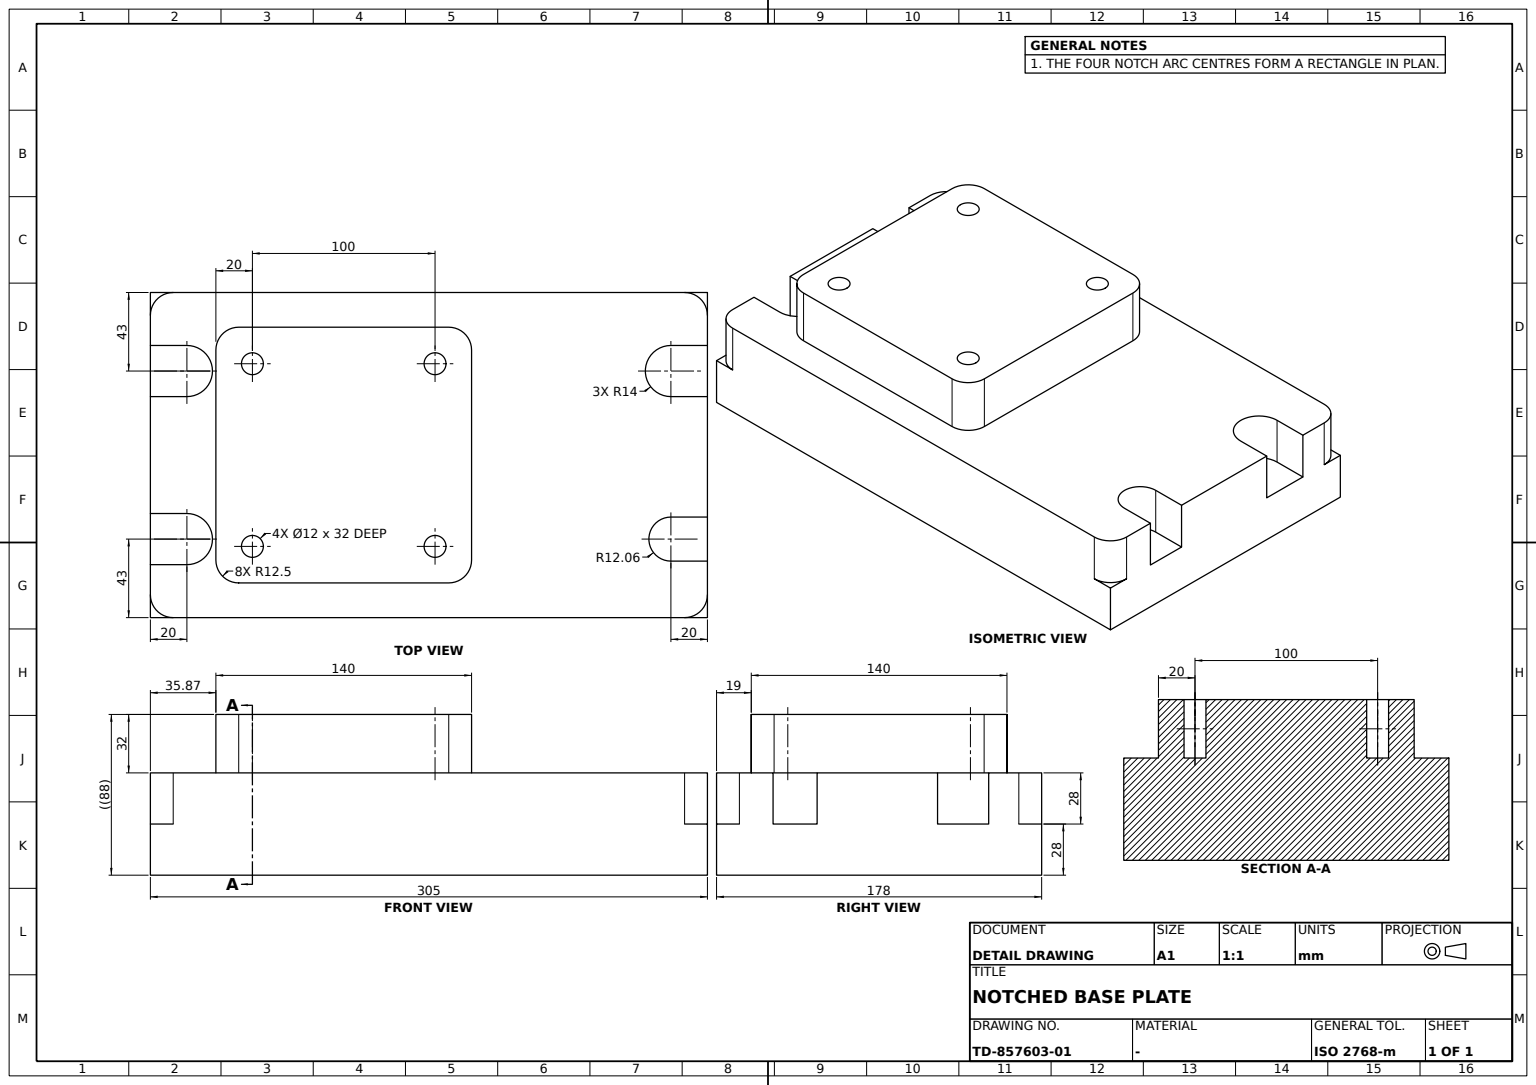
ISO-10303-21;
HEADER;
FILE_DESCRIPTION((''),'2;1');
FILE_NAME('','',(''),(''),'','','');
FILE_SCHEMA(('AUTOMOTIVE_DESIGN'));
ENDSEC;
DATA;
#1=APPLICATION_CONTEXT('');
#2=PRODUCT_CONTEXT('',#1,'mechanical');
#3=PRODUCT('','','',(#2));
#4=PRODUCT_DEFINITION_FORMATION('','',#3);
#5=PRODUCT_DEFINITION_CONTEXT('',#1,'design');
#6=PRODUCT_DEFINITION('','',#4,#5);
#7=PRODUCT_DEFINITION_SHAPE('','',#6);
#8=(LENGTH_UNIT()NAMED_UNIT(*)SI_UNIT(.MILLI.,.METRE.));
#9=(NAMED_UNIT(*)PLANE_ANGLE_UNIT()SI_UNIT($,.RADIAN.));
#10=(NAMED_UNIT(*)SI_UNIT($,.STERADIAN.)SOLID_ANGLE_UNIT());
#11=UNCERTAINTY_MEASURE_WITH_UNIT(LENGTH_MEASURE(1.E-05),#8,'distance_accuracy_value','');
#12=(GEOMETRIC_REPRESENTATION_CONTEXT(3)GLOBAL_UNCERTAINTY_ASSIGNED_CONTEXT((#11))GLOBAL_UNIT_ASSIGNED_CONTEXT((#8,#9,#10))REPRESENTATION_CONTEXT('',''));
#13=CARTESIAN_POINT('',(44.,50.,0.));
#14=VERTEX_POINT('',#13);
#15=CARTESIAN_POINT('',(56.,50.,0.));
#16=VERTEX_POINT('',#15);
#17=CARTESIAN_POINT('',(50.,50.,0.));
#18=DIRECTION('',(0.,0.,1.));
#19=DIRECTION('',(1.,0.,0.));
#20=AXIS2_PLACEMENT_3D('',#17,#18,#19);
#21=CIRCLE('',#20,6.);
#22=EDGE_CURVE('',#14,#16,#21,.T.);
#23=ORIENTED_EDGE('',*,*,#22,.F.);
#24=CARTESIAN_POINT('',(44.,50.,32.));
#25=VERTEX_POINT('',#24);
#26=CARTESIAN_POINT('',(44.,50.,16.));
#27=VECTOR('',#18,1000.);
#28=LINE('',#26,#27);
#29=EDGE_CURVE('',#14,#25,#28,.T.);
#30=ORIENTED_EDGE('',*,*,#29,.T.);
#31=CARTESIAN_POINT('',(56.,50.,32.));
#32=VERTEX_POINT('',#31);
#33=CARTESIAN_POINT('',(50.,50.,32.));
#34=AXIS2_PLACEMENT_3D('',#33,#18,#19);
#35=CIRCLE('',#34,6.);
#36=EDGE_CURVE('',#25,#32,#35,.T.);
#37=ORIENTED_EDGE('',*,*,#36,.T.);
#38=CARTESIAN_POINT('',(56.,50.,16.));
#39=LINE('',#38,#27);
#40=EDGE_CURVE('',#16,#32,#39,.T.);
#41=ORIENTED_EDGE('',*,*,#40,.F.);
#42=EDGE_LOOP('',(#23,#30,#37,#41));
#43=FACE_OUTER_BOUND('',#42,.T.);
#44=CARTESIAN_POINT('',(50.,50.,16.));
#45=DIRECTION('',(0.,0.,-1.));
#46=AXIS2_PLACEMENT_3D('',#44,#45,#19);
#47=CYLINDRICAL_SURFACE('',#46,6.);
#48=ADVANCED_FACE('',(#43),#47,.F.);
#49=EDGE_CURVE('',#16,#14,#21,.T.);
#50=ORIENTED_EDGE('',*,*,#49,.T.);
#51=ORIENTED_EDGE('',*,*,#22,.T.);
#52=EDGE_LOOP('',(#50,#51));
#53=FACE_BOUND('',#52,.T.);
#54=CARTESIAN_POINT('',(44.,-50.,0.));
#55=VERTEX_POINT('',#54);
#56=CARTESIAN_POINT('',(56.,-50.,0.));
#57=VERTEX_POINT('',#56);
#58=CARTESIAN_POINT('',(50.,-50.,0.));
#59=AXIS2_PLACEMENT_3D('',#58,#18,#19);
#60=CIRCLE('',#59,6.);
#61=EDGE_CURVE('',#55,#57,#60,.T.);
#62=ORIENTED_EDGE('',*,*,#61,.T.);
#63=EDGE_CURVE('',#57,#55,#60,.T.);
#64=ORIENTED_EDGE('',*,*,#63,.T.);
#65=EDGE_LOOP('',(#62,#64));
#66=FACE_BOUND('',#65,.T.);
#67=CARTESIAN_POINT('',(-44.,-50.,0.));
#68=VERTEX_POINT('',#67);
#69=CARTESIAN_POINT('',(-56.,-50.,0.));
#70=VERTEX_POINT('',#69);
#71=CARTESIAN_POINT('',(-50.,-50.,0.));
#72=AXIS2_PLACEMENT_3D('',#71,#18,#19);
#73=CIRCLE('',#72,6.);
#74=EDGE_CURVE('',#68,#70,#73,.T.);
#75=ORIENTED_EDGE('',*,*,#74,.T.);
#76=EDGE_CURVE('',#70,#68,#73,.T.);
#77=ORIENTED_EDGE('',*,*,#76,.T.);
#78=EDGE_LOOP('',(#75,#77));
#79=FACE_BOUND('',#78,.T.);
#80=CARTESIAN_POINT('',(-46.,0.,0.));
#81=VERTEX_POINT('',#80);
#82=CARTESIAN_POINT('',(46.,0.,0.));
#83=VERTEX_POINT('',#82);
#84=CARTESIAN_POINT('',(0.,0.,0.));
#85=AXIS2_PLACEMENT_3D('',#84,#18,#19);
#86=CIRCLE('',#85,46.);
#87=EDGE_CURVE('',#81,#83,#86,.T.);
#88=ORIENTED_EDGE('',*,*,#87,.T.);
#89=EDGE_CURVE('',#83,#81,#86,.T.);
#90=ORIENTED_EDGE('',*,*,#89,.T.);
#91=EDGE_LOOP('',(#88,#90));
#92=FACE_BOUND('',#91,.T.);
#93=CARTESIAN_POINT('',(-70.,57.5,0.));
#94=VERTEX_POINT('',#93);
#95=CARTESIAN_POINT('',(-70.,-57.5,0.));
#96=VERTEX_POINT('',#95);
#97=CARTESIAN_POINT('',(-70.,0.,0.));
#98=DIRECTION('',(0.,-1.,0.));
#99=VECTOR('',#98,1000.);
#100=LINE('',#97,#99);
#101=EDGE_CURVE('',#94,#96,#100,.T.);
#102=ORIENTED_EDGE('',*,*,#101,.F.);
#103=CARTESIAN_POINT('',(-57.5,70.,0.));
#104=VERTEX_POINT('',#103);
#105=CARTESIAN_POINT('',(-57.5,57.5,0.));
#106=AXIS2_PLACEMENT_3D('',#105,#18,#19);
#107=CIRCLE('',#106,12.5);
#108=EDGE_CURVE('',#104,#94,#107,.T.);
#109=ORIENTED_EDGE('',*,*,#108,.F.);
#110=CARTESIAN_POINT('',(57.5,70.,0.));
#111=VERTEX_POINT('',#110);
#112=CARTESIAN_POINT('',(0.,70.,0.));
#113=DIRECTION('',(-1.,0.,0.));
#114=VECTOR('',#113,1000.);
#115=LINE('',#112,#114);
#116=EDGE_CURVE('',#111,#104,#115,.T.);
#117=ORIENTED_EDGE('',*,*,#116,.F.);
#118=CARTESIAN_POINT('',(70.,57.5,0.));
#119=VERTEX_POINT('',#118);
#120=CARTESIAN_POINT('',(57.5,57.5,0.));
#121=AXIS2_PLACEMENT_3D('',#120,#18,#19);
#122=CIRCLE('',#121,12.5);
#123=EDGE_CURVE('',#119,#111,#122,.T.);
#124=ORIENTED_EDGE('',*,*,#123,.F.);
#125=CARTESIAN_POINT('',(70.,-57.5,0.));
#126=VERTEX_POINT('',#125);
#127=CARTESIAN_POINT('',(70.,0.,0.));
#128=DIRECTION('',(0.,1.,0.));
#129=VECTOR('',#128,1000.);
#130=LINE('',#127,#129);
#131=EDGE_CURVE('',#126,#119,#130,.T.);
#132=ORIENTED_EDGE('',*,*,#131,.F.);
#133=CARTESIAN_POINT('',(57.5,-70.,0.));
#134=VERTEX_POINT('',#133);
#135=CARTESIAN_POINT('',(57.5,-57.5,0.));
#136=AXIS2_PLACEMENT_3D('',#135,#18,#19);
#137=CIRCLE('',#136,12.5);
#138=EDGE_CURVE('',#134,#126,#137,.T.);
#139=ORIENTED_EDGE('',*,*,#138,.F.);
#140=CARTESIAN_POINT('',(-57.5,-70.,0.));
#141=VERTEX_POINT('',#140);
#142=CARTESIAN_POINT('',(0.,-70.,0.));
#143=VECTOR('',#19,1000.);
#144=LINE('',#142,#143);
#145=EDGE_CURVE('',#141,#134,#144,.T.);
#146=ORIENTED_EDGE('',*,*,#145,.F.);
#147=CARTESIAN_POINT('',(-57.5,-57.5,0.));
#148=AXIS2_PLACEMENT_3D('',#147,#18,#19);
#149=CIRCLE('',#148,12.5);
#150=EDGE_CURVE('',#96,#141,#149,.T.);
#151=ORIENTED_EDGE('',*,*,#150,.F.);
#152=EDGE_LOOP('',(#102,#109,#117,#124,#132,#139,#146,#151));
#153=FACE_OUTER_BOUND('',#152,.T.);
#154=CARTESIAN_POINT('',(-44.,50.,0.));
#155=VERTEX_POINT('',#154);
#156=CARTESIAN_POINT('',(-56.,50.,0.));
#157=VERTEX_POINT('',#156);
#158=CARTESIAN_POINT('',(-50.,50.,0.));
#159=AXIS2_PLACEMENT_3D('',#158,#18,#19);
#160=CIRCLE('',#159,6.);
#161=EDGE_CURVE('',#155,#157,#160,.T.);
#162=ORIENTED_EDGE('',*,*,#161,.T.);
#163=EDGE_CURVE('',#157,#155,#160,.T.);
#164=ORIENTED_EDGE('',*,*,#163,.T.);
#165=EDGE_LOOP('',(#162,#164));
#166=FACE_BOUND('',#165,.T.);
#167=PLANE('',#85);
#168=ADVANCED_FACE('',(#53,#66,#79,#92,#153,#166),#167,.F.);
#169=CARTESIAN_POINT('',(57.5,-70.,32.));
#170=VERTEX_POINT('',#169);
#171=CARTESIAN_POINT('',(57.5,-70.,16.));
#172=LINE('',#171,#27);
#173=EDGE_CURVE('',#134,#170,#172,.T.);
#174=ORIENTED_EDGE('',*,*,#173,.T.);
#175=CARTESIAN_POINT('',(-57.5,-70.,32.));
#176=VERTEX_POINT('',#175);
#177=CARTESIAN_POINT('',(0.,-70.,32.));
#178=LINE('',#177,#143);
#179=EDGE_CURVE('',#176,#170,#178,.T.);
#180=ORIENTED_EDGE('',*,*,#179,.F.);
#181=CARTESIAN_POINT('',(-57.5,-70.,16.));
#182=LINE('',#181,#27);
#183=EDGE_CURVE('',#141,#176,#182,.T.);
#184=ORIENTED_EDGE('',*,*,#183,.F.);
#185=ORIENTED_EDGE('',*,*,#145,.T.);
#186=EDGE_LOOP('',(#174,#180,#184,#185));
#187=FACE_OUTER_BOUND('',#186,.T.);
#188=CARTESIAN_POINT('',(70.,-70.,0.));
#189=AXIS2_PLACEMENT_3D('',#188,#128,#113);
#190=PLANE('',#189);
#191=ADVANCED_FACE('',(#187),#190,.F.);
#192=ORIENTED_EDGE('',*,*,#74,.F.);
#193=CARTESIAN_POINT('',(-44.,-50.,32.));
#194=VERTEX_POINT('',#193);
#195=CARTESIAN_POINT('',(-44.,-50.,16.));
#196=LINE('',#195,#27);
#197=EDGE_CURVE('',#68,#194,#196,.T.);
#198=ORIENTED_EDGE('',*,*,#197,.T.);
#199=CARTESIAN_POINT('',(-56.,-50.,32.));
#200=VERTEX_POINT('',#199);
#201=CARTESIAN_POINT('',(-50.,-50.,32.));
#202=AXIS2_PLACEMENT_3D('',#201,#18,#19);
#203=CIRCLE('',#202,6.);
#204=EDGE_CURVE('',#194,#200,#203,.T.);
#205=ORIENTED_EDGE('',*,*,#204,.T.);
#206=CARTESIAN_POINT('',(-56.,-50.,16.));
#207=LINE('',#206,#27);
#208=EDGE_CURVE('',#70,#200,#207,.T.);
#209=ORIENTED_EDGE('',*,*,#208,.F.);
#210=EDGE_LOOP('',(#192,#198,#205,#209));
#211=FACE_OUTER_BOUND('',#210,.T.);
#212=CARTESIAN_POINT('',(-50.,-50.,16.));
#213=AXIS2_PLACEMENT_3D('',#212,#45,#19);
#214=CYLINDRICAL_SURFACE('',#213,6.);
#215=ADVANCED_FACE('',(#211),#214,.F.);
#216=CARTESIAN_POINT('',(70.,-57.5,32.));
#217=VERTEX_POINT('',#216);
#218=CARTESIAN_POINT('',(57.5,-57.5,32.));
#219=AXIS2_PLACEMENT_3D('',#218,#45,#19);
#220=CIRCLE('',#219,12.5);
#221=EDGE_CURVE('',#217,#170,#220,.T.);
#222=ORIENTED_EDGE('',*,*,#221,.T.);
#223=ORIENTED_EDGE('',*,*,#173,.F.);
#224=ORIENTED_EDGE('',*,*,#138,.T.);
#225=CARTESIAN_POINT('',(70.,-57.5,16.));
#226=LINE('',#225,#27);
#227=EDGE_CURVE('',#126,#217,#226,.T.);
#228=ORIENTED_EDGE('',*,*,#227,.T.);
#229=EDGE_LOOP('',(#222,#223,#224,#228));
#230=FACE_OUTER_BOUND('',#229,.T.);
#231=CARTESIAN_POINT('',(57.5,-57.5,16.));
#232=AXIS2_PLACEMENT_3D('',#231,#45,#19);
#233=CYLINDRICAL_SURFACE('',#232,12.5);
#234=ADVANCED_FACE('',(#230),#233,.T.);
#235=ORIENTED_EDGE('',*,*,#101,.T.);
#236=CARTESIAN_POINT('',(-70.,-57.5,32.));
#237=VERTEX_POINT('',#236);
#238=CARTESIAN_POINT('',(-70.,-57.5,16.));
#239=LINE('',#238,#27);
#240=EDGE_CURVE('',#96,#237,#239,.T.);
#241=ORIENTED_EDGE('',*,*,#240,.T.);
#242=CARTESIAN_POINT('',(-70.,57.5,32.));
#243=VERTEX_POINT('',#242);
#244=CARTESIAN_POINT('',(-70.,0.,32.));
#245=LINE('',#244,#99);
#246=EDGE_CURVE('',#243,#237,#245,.T.);
#247=ORIENTED_EDGE('',*,*,#246,.F.);
#248=CARTESIAN_POINT('',(-70.,57.5,16.));
#249=LINE('',#248,#27);
#250=EDGE_CURVE('',#94,#243,#249,.T.);
#251=ORIENTED_EDGE('',*,*,#250,.F.);
#252=EDGE_LOOP('',(#235,#241,#247,#251));
#253=FACE_OUTER_BOUND('',#252,.T.);
#254=CARTESIAN_POINT('',(-70.,70.,0.));
#255=AXIS2_PLACEMENT_3D('',#254,#113,#98);
#256=PLANE('',#255);
#257=ADVANCED_FACE('',(#253),#256,.T.);
#258=EDGE_CURVE('',#32,#25,#35,.T.);
#259=ORIENTED_EDGE('',*,*,#258,.T.);
#260=ORIENTED_EDGE('',*,*,#29,.F.);
#261=ORIENTED_EDGE('',*,*,#49,.F.);
#262=ORIENTED_EDGE('',*,*,#40,.T.);
#263=EDGE_LOOP('',(#259,#260,#261,#262));
#264=FACE_OUTER_BOUND('',#263,.T.);
#265=ADVANCED_FACE('',(#264),#47,.F.);
#266=CARTESIAN_POINT('',(44.,-50.,32.));
#267=VERTEX_POINT('',#266);
#268=CARTESIAN_POINT('',(44.,-50.,16.));
#269=LINE('',#268,#27);
#270=EDGE_CURVE('',#55,#267,#269,.T.);
#271=ORIENTED_EDGE('',*,*,#270,.F.);
#272=ORIENTED_EDGE('',*,*,#63,.F.);
#273=CARTESIAN_POINT('',(56.,-50.,32.));
#274=VERTEX_POINT('',#273);
#275=CARTESIAN_POINT('',(56.,-50.,16.));
#276=LINE('',#275,#27);
#277=EDGE_CURVE('',#57,#274,#276,.T.);
#278=ORIENTED_EDGE('',*,*,#277,.T.);
#279=CARTESIAN_POINT('',(50.,-50.,32.));
#280=AXIS2_PLACEMENT_3D('',#279,#18,#19);
#281=CIRCLE('',#280,6.);
#282=EDGE_CURVE('',#274,#267,#281,.T.);
#283=ORIENTED_EDGE('',*,*,#282,.T.);
#284=EDGE_LOOP('',(#271,#272,#278,#283));
#285=FACE_OUTER_BOUND('',#284,.T.);
#286=CARTESIAN_POINT('',(50.,-50.,16.));
#287=AXIS2_PLACEMENT_3D('',#286,#45,#19);
#288=CYLINDRICAL_SURFACE('',#287,6.);
#289=ADVANCED_FACE('',(#285),#288,.F.);
#290=CARTESIAN_POINT('',(-46.,0.,32.));
#291=VERTEX_POINT('',#290);
#292=CARTESIAN_POINT('',(-46.,0.,15.34));
#293=VECTOR('',#45,1000.);
#294=LINE('',#292,#293);
#295=EDGE_CURVE('',#291,#81,#294,.T.);
#296=ORIENTED_EDGE('',*,*,#295,.T.);
#297=ORIENTED_EDGE('',*,*,#89,.F.);
#298=CARTESIAN_POINT('',(46.,0.,32.));
#299=VERTEX_POINT('',#298);
#300=CARTESIAN_POINT('',(46.,0.,15.34));
#301=LINE('',#300,#293);
#302=EDGE_CURVE('',#299,#83,#301,.T.);
#303=ORIENTED_EDGE('',*,*,#302,.F.);
#304=CARTESIAN_POINT('',(0.,0.,32.));
#305=AXIS2_PLACEMENT_3D('',#304,#18,#19);
#306=CIRCLE('',#305,46.);
#307=EDGE_CURVE('',#299,#291,#306,.T.);
#308=ORIENTED_EDGE('',*,*,#307,.T.);
#309=EDGE_LOOP('',(#296,#297,#303,#308));
#310=FACE_OUTER_BOUND('',#309,.T.);
#311=CARTESIAN_POINT('',(0.,0.,15.34));
#312=AXIS2_PLACEMENT_3D('',#311,#45,#19);
#313=CYLINDRICAL_SURFACE('',#312,46.);
#314=ADVANCED_FACE('',(#310),#313,.F.);
#315=ORIENTED_EDGE('',*,*,#61,.F.);
#316=ORIENTED_EDGE('',*,*,#270,.T.);
#317=EDGE_CURVE('',#267,#274,#281,.T.);
#318=ORIENTED_EDGE('',*,*,#317,.T.);
#319=ORIENTED_EDGE('',*,*,#277,.F.);
#320=EDGE_LOOP('',(#315,#316,#318,#319));
#321=FACE_OUTER_BOUND('',#320,.T.);
#322=ADVANCED_FACE('',(#321),#288,.F.);
#323=ORIENTED_EDGE('',*,*,#197,.F.);
#324=ORIENTED_EDGE('',*,*,#76,.F.);
#325=ORIENTED_EDGE('',*,*,#208,.T.);
#326=EDGE_CURVE('',#200,#194,#203,.T.);
#327=ORIENTED_EDGE('',*,*,#326,.T.);
#328=EDGE_LOOP('',(#323,#324,#325,#327));
#329=FACE_OUTER_BOUND('',#328,.T.);
#330=ADVANCED_FACE('',(#329),#214,.F.);
#331=ORIENTED_EDGE('',*,*,#161,.F.);
#332=CARTESIAN_POINT('',(-44.,50.,32.));
#333=VERTEX_POINT('',#332);
#334=CARTESIAN_POINT('',(-44.,50.,16.));
#335=LINE('',#334,#27);
#336=EDGE_CURVE('',#155,#333,#335,.T.);
#337=ORIENTED_EDGE('',*,*,#336,.T.);
#338=CARTESIAN_POINT('',(-56.,50.,32.));
#339=VERTEX_POINT('',#338);
#340=CARTESIAN_POINT('',(-50.,50.,32.));
#341=AXIS2_PLACEMENT_3D('',#340,#18,#19);
#342=CIRCLE('',#341,6.);
#343=EDGE_CURVE('',#333,#339,#342,.T.);
#344=ORIENTED_EDGE('',*,*,#343,.T.);
#345=CARTESIAN_POINT('',(-56.,50.,16.));
#346=LINE('',#345,#27);
#347=EDGE_CURVE('',#157,#339,#346,.T.);
#348=ORIENTED_EDGE('',*,*,#347,.F.);
#349=EDGE_LOOP('',(#331,#337,#344,#348));
#350=FACE_OUTER_BOUND('',#349,.T.);
#351=CARTESIAN_POINT('',(-50.,50.,16.));
#352=AXIS2_PLACEMENT_3D('',#351,#45,#19);
#353=CYLINDRICAL_SURFACE('',#352,6.);
#354=ADVANCED_FACE('',(#350),#353,.F.);
#355=CARTESIAN_POINT('',(57.5,70.,32.));
#356=VERTEX_POINT('',#355);
#357=CARTESIAN_POINT('',(57.5,70.,16.));
#358=LINE('',#357,#27);
#359=EDGE_CURVE('',#111,#356,#358,.T.);
#360=ORIENTED_EDGE('',*,*,#359,.T.);
#361=CARTESIAN_POINT('',(70.,57.5,32.));
#362=VERTEX_POINT('',#361);
#363=CARTESIAN_POINT('',(57.5,57.5,32.));
#364=AXIS2_PLACEMENT_3D('',#363,#45,#19);
#365=CIRCLE('',#364,12.5);
#366=EDGE_CURVE('',#356,#362,#365,.T.);
#367=ORIENTED_EDGE('',*,*,#366,.T.);
#368=CARTESIAN_POINT('',(70.,57.5,16.));
#369=LINE('',#368,#27);
#370=EDGE_CURVE('',#119,#362,#369,.T.);
#371=ORIENTED_EDGE('',*,*,#370,.F.);
#372=ORIENTED_EDGE('',*,*,#123,.T.);
#373=EDGE_LOOP('',(#360,#367,#371,#372));
#374=FACE_OUTER_BOUND('',#373,.T.);
#375=CARTESIAN_POINT('',(57.5,57.5,16.));
#376=AXIS2_PLACEMENT_3D('',#375,#45,#128);
#377=CYLINDRICAL_SURFACE('',#376,12.5);
#378=ADVANCED_FACE('',(#374),#377,.T.);
#379=CARTESIAN_POINT('',(-57.5,70.,32.));
#380=VERTEX_POINT('',#379);
#381=CARTESIAN_POINT('',(-57.5,57.5,32.));
#382=AXIS2_PLACEMENT_3D('',#381,#45,#19);
#383=CIRCLE('',#382,12.5);
#384=EDGE_CURVE('',#243,#380,#383,.T.);
#385=ORIENTED_EDGE('',*,*,#384,.T.);
#386=CARTESIAN_POINT('',(-57.5,70.,16.));
#387=LINE('',#386,#27);
#388=EDGE_CURVE('',#104,#380,#387,.T.);
#389=ORIENTED_EDGE('',*,*,#388,.F.);
#390=ORIENTED_EDGE('',*,*,#108,.T.);
#391=ORIENTED_EDGE('',*,*,#250,.T.);
#392=EDGE_LOOP('',(#385,#389,#390,#391));
#393=FACE_OUTER_BOUND('',#392,.T.);
#394=CARTESIAN_POINT('',(-57.5,57.5,16.));
#395=AXIS2_PLACEMENT_3D('',#394,#45,#113);
#396=CYLINDRICAL_SURFACE('',#395,12.5);
#397=ADVANCED_FACE('',(#393),#396,.T.);
#398=ORIENTED_EDGE('',*,*,#359,.F.);
#399=ORIENTED_EDGE('',*,*,#116,.T.);
#400=ORIENTED_EDGE('',*,*,#388,.T.);
#401=CARTESIAN_POINT('',(0.,70.,32.));
#402=LINE('',#401,#114);
#403=EDGE_CURVE('',#356,#380,#402,.T.);
#404=ORIENTED_EDGE('',*,*,#403,.F.);
#405=EDGE_LOOP('',(#398,#399,#400,#404));
#406=FACE_OUTER_BOUND('',#405,.T.);
#407=AXIS2_PLACEMENT_3D('',#254,#98,#19);
#408=PLANE('',#407);
#409=ADVANCED_FACE('',(#406),#408,.F.);
#410=CARTESIAN_POINT('',(-57.5,-57.5,32.));
#411=AXIS2_PLACEMENT_3D('',#410,#45,#19);
#412=CIRCLE('',#411,12.5);
#413=EDGE_CURVE('',#176,#237,#412,.T.);
#414=ORIENTED_EDGE('',*,*,#413,.T.);
#415=ORIENTED_EDGE('',*,*,#240,.F.);
#416=ORIENTED_EDGE('',*,*,#150,.T.);
#417=ORIENTED_EDGE('',*,*,#183,.T.);
#418=EDGE_LOOP('',(#414,#415,#416,#417));
#419=FACE_OUTER_BOUND('',#418,.T.);
#420=CARTESIAN_POINT('',(-57.5,-57.5,16.));
#421=AXIS2_PLACEMENT_3D('',#420,#45,#98);
#422=CYLINDRICAL_SURFACE('',#421,12.5);
#423=ADVANCED_FACE('',(#419),#422,.T.);
#424=ORIENTED_EDGE('',*,*,#36,.F.);
#425=ORIENTED_EDGE('',*,*,#258,.F.);
#426=EDGE_LOOP('',(#424,#425));
#427=FACE_BOUND('',#426,.T.);
#428=ORIENTED_EDGE('',*,*,#307,.F.);
#429=EDGE_CURVE('',#291,#299,#306,.T.);
#430=ORIENTED_EDGE('',*,*,#429,.F.);
#431=EDGE_LOOP('',(#428,#430));
#432=FACE_BOUND('',#431,.T.);
#433=ORIENTED_EDGE('',*,*,#326,.F.);
#434=ORIENTED_EDGE('',*,*,#204,.F.);
#435=EDGE_LOOP('',(#433,#434));
#436=FACE_BOUND('',#435,.T.);
#437=ORIENTED_EDGE('',*,*,#317,.F.);
#438=ORIENTED_EDGE('',*,*,#282,.F.);
#439=EDGE_LOOP('',(#437,#438));
#440=FACE_BOUND('',#439,.T.);
#441=EDGE_CURVE('',#339,#333,#342,.T.);
#442=ORIENTED_EDGE('',*,*,#441,.F.);
#443=ORIENTED_EDGE('',*,*,#343,.F.);
#444=EDGE_LOOP('',(#442,#443));
#445=FACE_BOUND('',#444,.T.);
#446=CARTESIAN_POINT('',(70.,0.,32.));
#447=LINE('',#446,#129);
#448=EDGE_CURVE('',#217,#362,#447,.T.);
#449=ORIENTED_EDGE('',*,*,#448,.T.);
#450=ORIENTED_EDGE('',*,*,#366,.F.);
#451=ORIENTED_EDGE('',*,*,#403,.T.);
#452=ORIENTED_EDGE('',*,*,#384,.F.);
#453=ORIENTED_EDGE('',*,*,#246,.T.);
#454=ORIENTED_EDGE('',*,*,#413,.F.);
#455=ORIENTED_EDGE('',*,*,#179,.T.);
#456=ORIENTED_EDGE('',*,*,#221,.F.);
#457=EDGE_LOOP('',(#449,#450,#451,#452,#453,#454,#455,#456));
#458=FACE_OUTER_BOUND('',#457,.T.);
#459=PLANE('',#305);
#460=ADVANCED_FACE('',(#427,#432,#436,#440,#445,#458),#459,.T.);
#461=ORIENTED_EDGE('',*,*,#87,.F.);
#462=ORIENTED_EDGE('',*,*,#295,.F.);
#463=ORIENTED_EDGE('',*,*,#429,.T.);
#464=ORIENTED_EDGE('',*,*,#302,.T.);
#465=EDGE_LOOP('',(#461,#462,#463,#464));
#466=FACE_OUTER_BOUND('',#465,.T.);
#467=ADVANCED_FACE('',(#466),#313,.F.);
#468=ORIENTED_EDGE('',*,*,#347,.T.);
#469=ORIENTED_EDGE('',*,*,#441,.T.);
#470=ORIENTED_EDGE('',*,*,#336,.F.);
#471=ORIENTED_EDGE('',*,*,#163,.F.);
#472=EDGE_LOOP('',(#468,#469,#470,#471));
#473=FACE_OUTER_BOUND('',#472,.T.);
#474=ADVANCED_FACE('',(#473),#353,.F.);
#475=ORIENTED_EDGE('',*,*,#370,.T.);
#476=ORIENTED_EDGE('',*,*,#448,.F.);
#477=ORIENTED_EDGE('',*,*,#227,.F.);
#478=ORIENTED_EDGE('',*,*,#131,.T.);
#479=EDGE_LOOP('',(#475,#476,#477,#478));
#480=FACE_OUTER_BOUND('',#479,.T.);
#481=AXIS2_PLACEMENT_3D('',#188,#19,#128);
#482=PLANE('',#481);
#483=ADVANCED_FACE('',(#480),#482,.T.);
#484=CLOSED_SHELL('',(#48,#168,#191,#215,#234,#257,#265,#289,#314,#322,#330,#354,#378,#397,#409,#423,#460,#467,#474,#483));
#485=MANIFOLD_SOLID_BREP('',#484);
#486=ADVANCED_BREP_SHAPE_REPRESENTATION('',(#485),#12);
#487=SHAPE_DEFINITION_REPRESENTATION(#7,#486);
ENDSEC;
END-ISO-10303-21;
